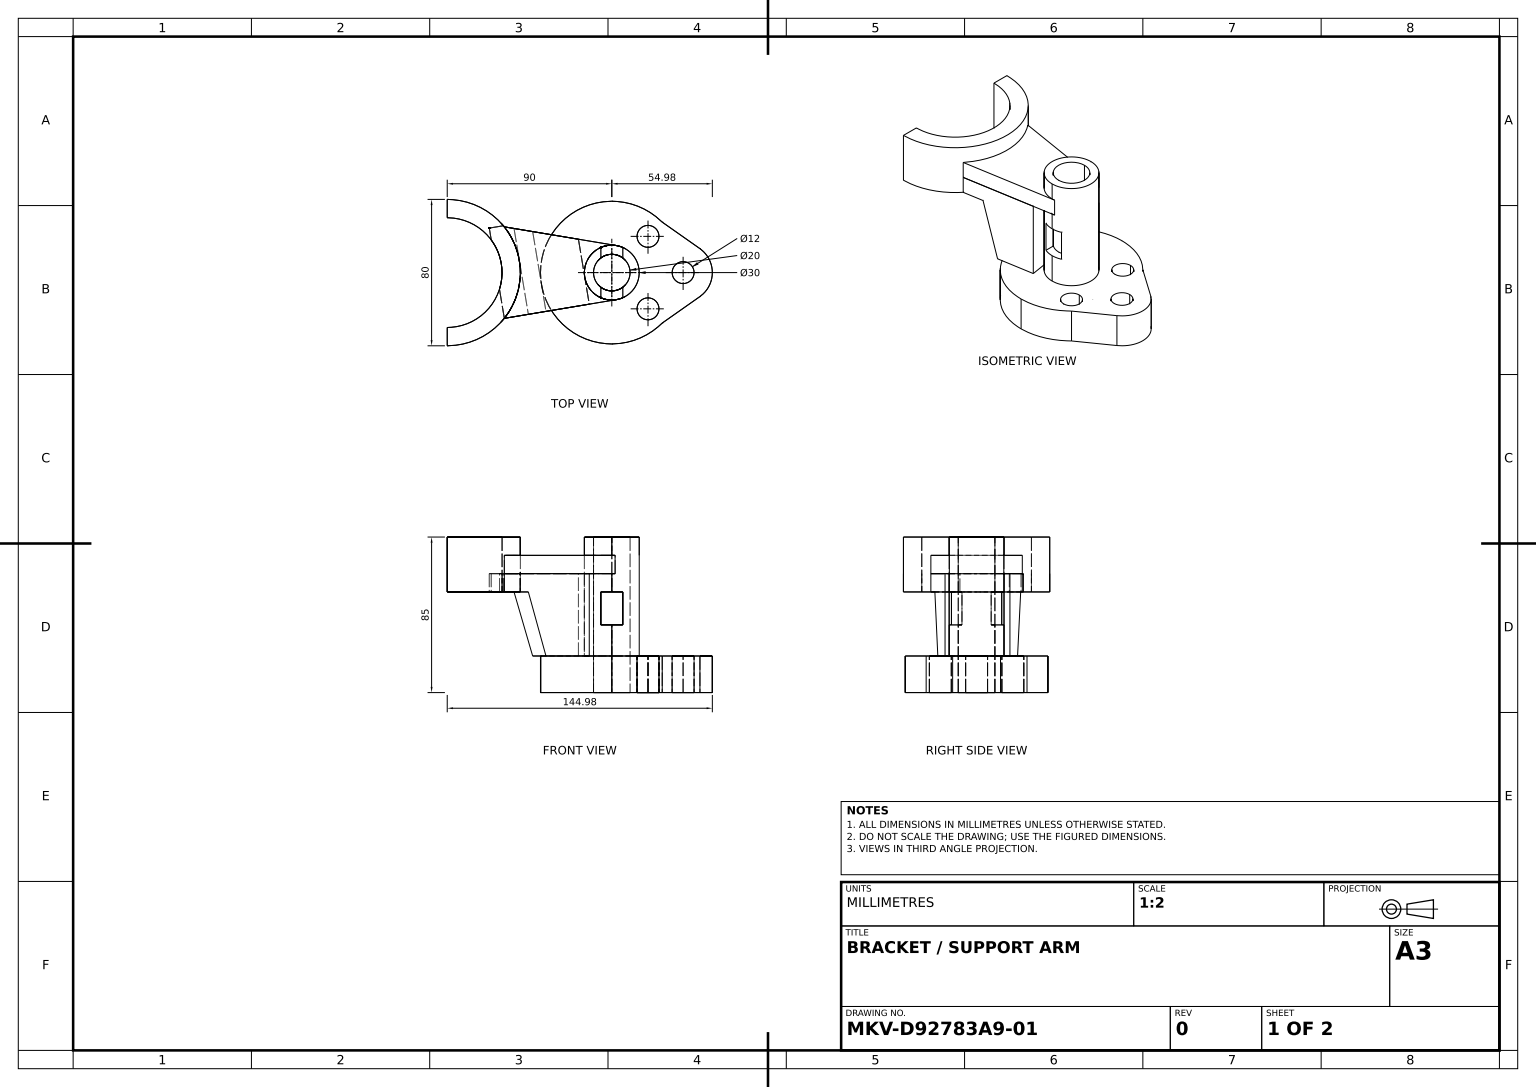
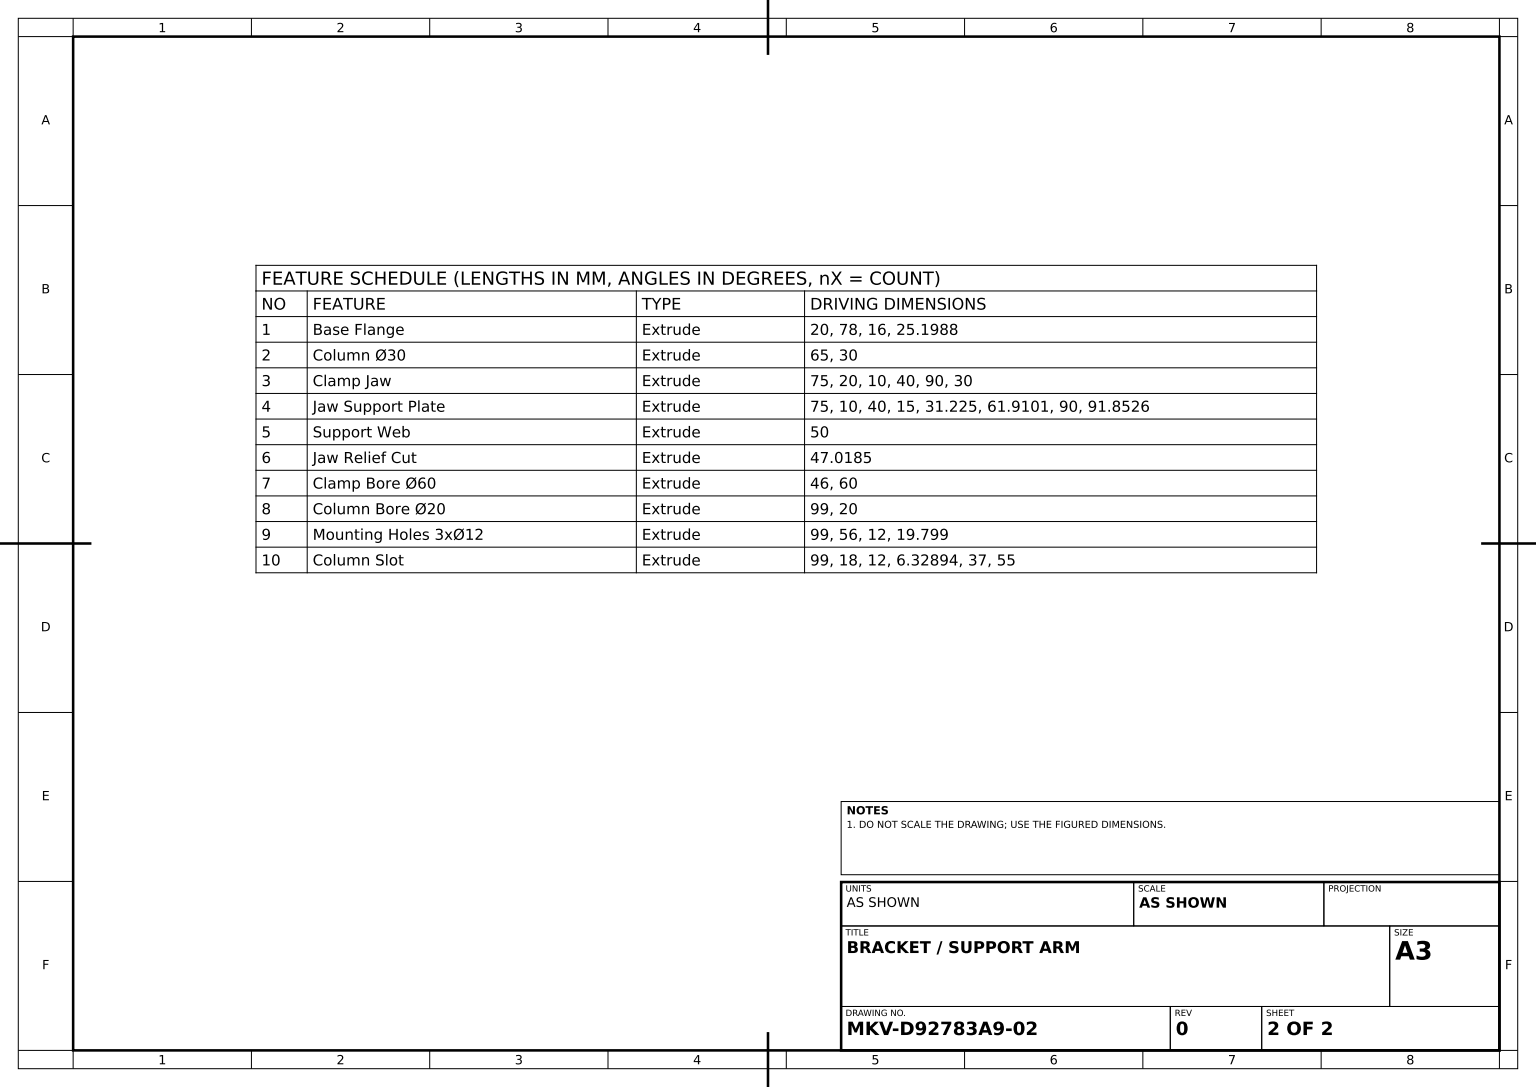
solid
v1 (-18.251094,65,-18.239168)
v2 (-12.328937,65,17.249284)
e1 v1 v2 LINE
v3 (-58.77501,65,-25)
e2 v3 v1 LINE
v4 (-59.272054,65,-25.608462)
e3 v3 v4 CIRCLE(AX(P(-90,65,0),D(0,1,0),D(0,0,1)),40)
v5 (-67.004985,65,-24.318024)
e4 v5 v4 LINE
v6 (-65.936474,65,-17.914985)
e5 v5 v6 LINE
v7 (-61.423225,65,9.130604)
e6 v6 v7 CIRCLE(AX(P(-90,65,0),D(0,-1,0),D(0,0,-1)),30)
v8 (-58.77501,65,25)
e7 v7 v8 LINE
e8 v8 v2 LINE
face PLANE(AX(P(-5.763505,65,-34.537733),D(0,-1,0),D(0,0,-1))) rev [-e1 -e2 e3 -e4 e5 e6 e7 e8]
v9 (-65.936474,55,-17.914985)
e9 v6 v9 LINE
v10 (-61.423225,55,9.130604)
e10 v9 v10 CIRCLE(AX(P(-90,55,0),D(0,-1,0),D(0,0,-1)),30)
e11 v10 v7 LINE
face CYL(AX(P(-90,39,0),D(0,1,0),D(0,0,1)),30) rev [-e6 e9 e10 e11]
v11 (-67.004985,55,-24.318024)
v12 (-59.272054,55,-25.608462)
e12 v11 v12 LINE
e13 v5 v11 LINE
e14 v12 v4 LINE
face PLANE(AX(P(-5.763505,0,-34.537733),D(0.16459949,0,0.986360486),D(0.986360486,0,-0.16459949))) rev [-e12 -e13 e4 -e14]
v13 (-58.77501,55,25)
v14 (-45.640741,55,22.808211)
e15 v13 v14 LINE
e16 v10 v13 LINE
e17 v11 v9 LINE
v15 (-58.77501,55,-25)
e18 v12 v15 CIRCLE(AX(P(-90,55,0),D(0,-1,0),D(0,0,-1)),40)
v16 (-53.4711,55,-24.115119)
e19 v16 v15 LINE
e20 v16 v14 LINE
face PLANE(AX(P(-5.763505,55,-34.537733),D(0,-1,0),D(0,0,-1))) [-e15 -e16 -e10 -e17 e12 e18 -e19 e20]
e21 v15 v3 LINE
face CYL(AX(P(-90,20,0),D(0,1,0),D(0,0,1)),40) [-e21 -e18 e14 -e3]
v17 (-18.251094,20,-18.239168)
e22 v17 v1 LINE
v18 (-43.279787,20,-22.414845)
e23 v18 v17 LINE
e24 v16 v18 LINE
face PLANE(AX(P(2.466292,20,-14.78277),D(-0.164561124,0,0.986366887),D(0.986366887,0,0.164561124))) rev [-e22 -e23 -e24 e19 e21 e2]
v19 (-12.328937,20,17.249284)
e25 v17 v19 LINE
v20 (-36.001589,20,21.199672)
e26 v19 v20 LINE
e27 v18 v20 LINE
face PLANE(AX(P(-5.763505,20,-34.537733),D(0,1,0),D(-1,0,0))) rev [e23 e25 e26 -e27]
e28 v8 v13 LINE
e29 v20 v14 LINE
e30 v2 v19 LINE
face PLANE(AX(P(2.46647,0,14.780292),D(0.16459949,0,0.986360486),D(0.986360486,0,-0.16459949))) [-e8 e28 e15 -e29 -e26 -e30]
face PLANE(AX(P(-36.33976,-8.655333,-29.435302),D(0.950023612,0.268926666,-0.158535753),D(-0.272371281,0.962192229,0))) rev [-e20 e24 e27 e29]
face PLANE(AX(P(-67.004985,0,-24.318024),D(-0.986360486,0,0.16459949),D(0.16459949,0,0.986360486))) [-e11 e16 -e28 -e7]
face PLANE(AX(P(-67.004985,0,-24.318024),D(-0.986360486,0,0.16459949),D(0.16459949,0,0.986360486))) [-e5 e13 e17 -e9]
face PLANE(AX(P(-20.558912,0,-32.06874),D(-0.986360486,0,0.16459949),D(0.16459949,0,0.986360486))) rev [e1 e30 -e25 e22]
solid
v21 (-6,37,13.747727)
v22 (-6,55,13.747727)
e31 v21 v22 LINE
v23 (-6,37,8)
e32 v23 v21 LINE
v24 (-6,55,8)
e33 v24 v23 LINE
e34 v24 v22 LINE
face PLANE(AX(P(-6,37,-49.5),D(-1,0,0),D(0,0,1))) rev [-e31 -e32 -e33 e34]
v25 (39,0,-6)
v26 (39,0,6)
e35 v25 v26 CIRCLE(AX(P(39,0,0),D(0,1,0),D(0,0,1)),6)
v27 (39,20,-6)
e36 v25 v27 LINE
v28 (39,20,6)
e37 v27 v28 CIRCLE(AX(P(39,20,0),D(0,1,0),D(0,0,1)),6)
e38 v26 v28 LINE
face CYL(AX(P(39,-79,0),D(0,1,0),D(0,0,1)),6) rev [-e35 e36 e37 -e38]
v29 (-90,55,30)
v30 (-90,55,40)
e39 v29 v30 LINE
v31 (-90,55,-30)
e40 v31 v29 CIRCLE(AX(P(-90,55,0),D(0,-1,0),D(0,0,1)),30)
v32 (-90,55,-40)
e41 v32 v31 LINE
e42 v30 v32 CIRCLE(AX(P(-90,55,0),D(0,1,0),D(0,0,1)),40)
face PLANE(AX(P(-90,55,0),D(0,1,0),D(0,0,1))) rev [-e39 -e40 -e41 -e42]
v33 (-90,85,40)
e43 v33 v30 LINE
v34 (-90,85,-40)
e44 v34 v32 LINE
e45 v33 v34 CIRCLE(AX(P(-90,85,0),D(0,1,0),D(0,0,1)),40)
v35 (-58.77501,65,25)
v36 (-58.77501,65,-25)
e46 v35 v36 CIRCLE(AX(P(-90,65,0),D(0,1,0),D(0,0,1)),40)
v37 (-58.77501,75,25)
e47 v35 v37 LINE
v38 (-58.77501,75,-25)
e48 v37 v38 CIRCLE(AX(P(-90,75,0),D(0,1,0),D(0,0,1)),40)
e49 v36 v38 LINE
face CYL(AX(P(-90,85,0),D(0,-1,0),D(0,0,-1)),40) [e43 e42 -e44 -e45] [-e46 e47 e48 -e49]
v39 (6,37,8)
v40 (6,55,8)
e50 v39 v40 LINE
v41 (6,37,13.747727)
e51 v39 v41 LINE
v42 (6,55,13.747727)
e52 v42 v41 LINE
e53 v40 v42 LINE
face PLANE(AX(P(6,55,-49.5),D(1,0,0),D(0,1,0))) rev [-e50 e51 -e52 -e53]
v43 (-90,85,-30)
e54 v34 v43 LINE
e55 v43 v31 LINE
face PLANE(AX(P(-90,85,-30),D(1,0,0),D(0,0,-1))) rev [-e54 e44 e41 -e55]
v44 (1.79785,65,14.891868)
e56 v35 v44 LINE
v45 (1.852586,65,-14.885158)
e57 v36 v45 LINE
v46 (0,65,-15)
e58 v45 v46 CIRCLE(AX(P(0,65,0),D(0,1,0),D(0,0,1)),15)
v47 (0,65,15)
e59 v46 v47 CIRCLE(AX(P(0,65,0),D(0,1,0),D(0,0,1)),15)
e60 v47 v44 CIRCLE(AX(P(0,65,0),D(0,1,0),D(0,0,1)),15)
face PLANE(AX(P(0,65,0),D(0,1,0),D(0,0,1))) rev [-e56 e46 e57 e58 e59 e60]
v48 (-90,85,30)
e61 v43 v48 CIRCLE(AX(P(-90,85,0),D(0,-1,0),D(0,0,1)),30)
e62 v48 v33 LINE
face PLANE(AX(P(-90,85,0),D(0,1,0),D(0,0,1))) [e61 e62 e45 e54]
v49 (0,37,-10)
v50 (-6,37,-8)
e63 v49 v50 CIRCLE(AX(P(0,37,0),D(0,1,0),D(0,0,-1)),10)
v51 (6,37,-8)
e64 v51 v49 CIRCLE(AX(P(0,37,0),D(0,1,0),D(0,0,-1)),10)
v52 (6,37,-13.747727)
e65 v52 v51 LINE
v53 (0,37,-15)
e66 v53 v52 CIRCLE(AX(P(0,37,0),D(0,-1,0),D(0,0,-1)),15)
v54 (-6,37,-13.747727)
e67 v54 v53 CIRCLE(AX(P(0,37,0),D(0,-1,0),D(0,0,-1)),15)
e68 v54 v50 LINE
face PLANE(AX(P(6,37,-49.5),D(0,-1,0),D(0,0,-1))) rev [-e63 -e64 -e65 -e66 -e67 e68]
v55 (27.577164,0,27.577164)
v56 (48.196998,0,13.092564)
e69 v55 v56 LINE
v57 (0,0,39)
e70 v57 v55 CIRCLE(AX(P(0,0,0),D(0,1,0),D(0,0,1)),39)
v58 (0,0,-39)
e71 v58 v57 CIRCLE(AX(P(0,0,0),D(0,1,0),D(0,0,1)),39)
v59 (27.577164,0,-27.577164)
e72 v59 v58 CIRCLE(AX(P(0,0,0),D(0,1,0),D(0,0,1)),39)
v60 (48.196998,0,-13.092564)
e73 v60 v59 LINE
e74 v56 v60 CIRCLE(AX(P(39,0,0),D(0,1,0),D(0,0,1)),16)
v61 (19.79899,0,-13.79899)
v62 (19.79899,0,-25.79899)
e75 v61 v62 CIRCLE(AX(P(19.79899,0,-19.79899),D(0,1,0),D(0,0,1)),6)
e76 v62 v61 CIRCLE(AX(P(19.79899,0,-19.79899),D(0,1,0),D(0,0,1)),6)
e77 v26 v25 CIRCLE(AX(P(39,0,0),D(0,1,0),D(0,0,1)),6)
v63 (19.79899,0,25.79899)
v64 (19.79899,0,13.79899)
e78 v63 v64 CIRCLE(AX(P(19.79899,0,19.79899),D(0,1,0),D(0,0,1)),6)
e79 v64 v63 CIRCLE(AX(P(19.79899,0,19.79899),D(0,1,0),D(0,0,1)),6)
v65 (0,0,-10)
v66 (0,0,10)
e80 v65 v66 CIRCLE(AX(P(0,0,0),D(0,1,0),D(0,0,1)),10)
e81 v66 v65 CIRCLE(AX(P(0,0,0),D(0,1,0),D(0,0,1)),10)
face PLANE(AX(P(39,0,0),D(0,1,0),D(0,0,1))) rev [-e69 -e70 -e71 -e72 -e73 -e74] [e75 e76] [e77 e35] [e78 e79] [e80 e81]
v67 (0,37,15)
v68 (0,20,15)
e82 v67 v68 LINE
e83 v67 v21 CIRCLE(AX(P(0,37,0),D(0,-1,0),D(0,0,-1)),15)
v69 (0,55,15)
e84 v22 v69 CIRCLE(AX(P(0,55,0),D(0,1,0),D(0,0,1)),15)
e85 v47 v69 LINE
v70 (0,55,-15)
e86 v46 v70 LINE
v71 (-6,55,-13.747727)
e87 v70 v71 CIRCLE(AX(P(0,55,0),D(0,1,0),D(0,0,1)),15)
e88 v71 v54 LINE
v72 (0,20,-15)
e89 v53 v72 LINE
e90 v72 v68 CIRCLE(AX(P(0,20,0),D(0,1,0),D(0,0,1)),15)
face CYL(AX(P(0,85,0),D(0,-1,0),D(0,0,-1)),15) [-e82 e83 e31 e84 -e85 -e59 e86 e87 e88 e67 e89 e90]
v73 (1.852586,75,-14.885158)
e91 v38 v73 LINE
e92 v45 v73 LINE
face PLANE(AX(P(2.466292,65,-14.78277),D(-0.164561124,0,0.986366887),D(0.986366887,0,0.164561124))) rev [e49 e91 -e92 -e57]
v74 (19.79899,20,-13.79899)
e93 v61 v74 LINE
v75 (19.79899,20,-25.79899)
e94 v74 v75 CIRCLE(AX(P(19.79899,20,-19.79899),D(0,1,0),D(0,0,1)),6)
e95 v62 v75 LINE
face CYL(AX(P(19.79899,-79,-19.79899),D(0,1,0),D(0,0,1)),6) rev [e93 e94 -e95 -e75]
v76 (6,55,-13.747727)
e96 v76 v70 CIRCLE(AX(P(0,55,0),D(0,1,0),D(0,0,1)),15)
v77 (6,55,-8)
e97 v76 v77 LINE
v78 (0,55,-10)
e98 v78 v77 CIRCLE(AX(P(0,55,0),D(0,-1,0),D(0,0,1)),10)
v79 (-6,55,-8)
e99 v79 v78 CIRCLE(AX(P(0,55,0),D(0,-1,0),D(0,0,1)),10)
e100 v71 v79 LINE
face PLANE(AX(P(0,55,-49.5),D(0,1,0),D(0,0,1))) rev [-e87 -e96 e97 -e98 -e99 -e100]
v80 (0,85,10)
v81 (0,85,-10)
e101 v80 v81 CIRCLE(AX(P(0,85,0),D(0,1,0),D(0,0,1)),10)
e102 v81 v80 CIRCLE(AX(P(0,85,0),D(0,1,0),D(0,0,1)),10)
v82 (0,85,-15)
v83 (0,85,15)
e103 v82 v83 CIRCLE(AX(P(0,85,0),D(0,1,0),D(0,0,1)),15)
e104 v83 v82 CIRCLE(AX(P(0,85,0),D(0,1,0),D(0,0,1)),15)
face PLANE(AX(P(0,85,0),D(0,1,0),D(0,0,1))) [-e101 -e102] [e103 e104]
e105 v50 v79 LINE
e106 v78 v81 LINE
v84 (0,55,10)
e107 v84 v80 LINE
e108 v84 v24 CIRCLE(AX(P(0,55,0),D(0,-1,0),D(0,0,1)),10)
v85 (0,37,10)
e109 v23 v85 CIRCLE(AX(P(0,37,0),D(0,1,0),D(0,0,-1)),10)
e110 v66 v85 LINE
e111 v65 v49 LINE
face CYL(AX(P(0,-14,0),D(0,1,0),D(0,0,1)),10) rev [e105 e99 e106 e102 -e107 e108 e33 e109 -e110 -e80 e111 e63]
v86 (0,75,-15)
e112 v73 v86 CIRCLE(AX(P(0,75,0),D(0,1,0),D(0,0,1)),15)
e113 v82 v86 LINE
v87 (0,75,15)
e114 v83 v87 LINE
v88 (1.79785,75,14.891868)
e115 v87 v88 CIRCLE(AX(P(0,75,0),D(0,1,0),D(0,0,1)),15)
e116 v44 v88 LINE
e117 v69 v42 CIRCLE(AX(P(0,55,0),D(0,1,0),D(0,0,1)),15)
e118 v41 v67 CIRCLE(AX(P(0,37,0),D(0,-1,0),D(0,0,-1)),15)
e119 v68 v72 CIRCLE(AX(P(0,20,0),D(0,1,0),D(0,0,1)),15)
e120 v52 v76 LINE
face CYL(AX(P(0,85,0),D(0,-1,0),D(0,0,-1)),15) [e96 -e86 -e58 e92 e112 -e113 -e104 e114 e115 -e116 -e60 e85 e117 e52 e118 e82 e119 -e89 e66 e120]
e121 v48 v29 LINE
face CYL(AX(P(-90,85,0),D(0,-1,0),D(0,0,-1)),30) rev [e40 -e121 -e61 e55]
v89 (27.577164,20,27.577164)
e122 v89 v55 LINE
v90 (48.196998,20,13.092564)
e123 v90 v56 LINE
e124 v89 v90 LINE
face PLANE(AX(P(27.577164,20,27.577164),D(-0.574812356,0,-0.818285253),D(-0.818285253,0,0.574812356))) rev [e122 e69 -e123 -e124]
v91 (0,20,39)
e125 v91 v57 LINE
v92 (0,20,-39)
e126 v92 v91 CIRCLE(AX(P(0,20,0),D(0,1,0),D(0,0,1)),39)
e127 v92 v58 LINE
face CYL(AX(P(0,20,0),D(0,-1,0),D(0,0,-1)),39) [e71 -e125 -e126 e127]
e128 v91 v89 CIRCLE(AX(P(0,20,0),D(0,1,0),D(0,0,1)),39)
face CYL(AX(P(0,20,0),D(0,-1,0),D(0,0,-1)),39) [-e128 e125 e70 -e122]
e129 v75 v74 CIRCLE(AX(P(19.79899,20,-19.79899),D(0,1,0),D(0,0,1)),6)
face CYL(AX(P(19.79899,-79,-19.79899),D(0,1,0),D(0,0,1)),6) rev [-e76 e95 e129 -e93]
e130 v37 v88 LINE
face PLANE(AX(P(2.46647,65,14.780292),D(0.16459949,0,0.986360486),D(0.986360486,0,-0.16459949))) [-e130 -e47 e56 e116]
v93 (19.79899,20,13.79899)
e131 v64 v93 LINE
v94 (19.79899,20,25.79899)
e132 v63 v94 LINE
e133 v94 v93 CIRCLE(AX(P(19.79899,20,19.79899),D(0,1,0),D(0,0,1)),6)
face CYL(AX(P(19.79899,-79,19.79899),D(0,1,0),D(0,0,1)),6) rev [-e131 -e78 e132 e133]
e134 v86 v87 CIRCLE(AX(P(0,75,0),D(0,1,0),D(0,0,1)),15)
face CYL(AX(P(0,85,0),D(0,-1,0),D(0,0,-1)),15) [e113 e134 -e114 -e103]
face PLANE(AX(P(-6,37,-49.5),D(-1,0,0),D(0,0,1))) rev [e100 -e105 -e68 -e88]
e135 v77 v51 LINE
e136 v85 v39 CIRCLE(AX(P(0,37,0),D(0,1,0),D(0,0,-1)),10)
e137 v40 v84 CIRCLE(AX(P(0,55,0),D(0,-1,0),D(0,0,1)),10)
face CYL(AX(P(0,-14,0),D(0,1,0),D(0,0,1)),10) rev [e98 e135 e64 -e111 -e81 e110 e136 e50 e137 e107 e101 -e106]
face PLANE(AX(P(-90,85,30),D(1,0,0),D(0,0,-1))) rev [-e43 -e62 e121 e39]
face PLANE(AX(P(6,55,-49.5),D(1,0,0),D(0,1,0))) rev [-e135 -e97 -e120 e65]
face PLANE(AX(P(6,37,-49.5),D(0,-1,0),D(0,0,-1))) rev [-e109 e32 -e83 -e118 -e51 -e136]
face PLANE(AX(P(0,55,-49.5),D(0,1,0),D(0,0,1))) rev [e53 -e117 -e84 -e34 -e108 -e137]
e138 v93 v94 CIRCLE(AX(P(19.79899,20,19.79899),D(0,1,0),D(0,0,1)),6)
face CYL(AX(P(19.79899,-79,19.79899),D(0,1,0),D(0,0,1)),6) rev [e138 -e132 -e79 e131]
v95 (27.577164,20,-27.577164)
e139 v95 v92 CIRCLE(AX(P(0,20,0),D(0,1,0),D(0,0,1)),39)
v96 (48.196998,20,-13.092564)
e140 v90 v96 CIRCLE(AX(P(39,20,0),D(0,1,0),D(0,0,1)),16)
e141 v96 v95 LINE
e142 v28 v27 CIRCLE(AX(P(39,20,0),D(0,1,0),D(0,0,1)),6)
face PLANE(AX(P(39,20,0),D(0,1,0),D(0,0,1))) [e139 e126 e128 e124 e140 e141] [-e129 -e94] [-e133 -e138] [-e37 -e142] [-e90 -e119]
face CYL(AX(P(39,-79,0),D(0,1,0),D(0,0,1)),6) rev [-e36 -e77 e38 e142]
face PLANE(AX(P(0,75,0),D(0,1,0),D(0,0,1))) [-e134 -e112 -e91 -e48 e130 -e115]
e143 v95 v59 LINE
e144 v96 v60 LINE
face PLANE(AX(P(48.196998,20,-13.092564),D(-0.574812356,0,0.818285253),D(0.818285253,0,0.574812356))) rev [-e143 -e141 e144 e73]
face CYL(AX(P(39,20,0),D(0,-1,0),D(0,0,-1)),16) [e123 e74 -e144 -e140]
face CYL(AX(P(0,20,0),D(0,-1,0),D(0,0,-1)),39) [-e139 e143 e72 -e127]
